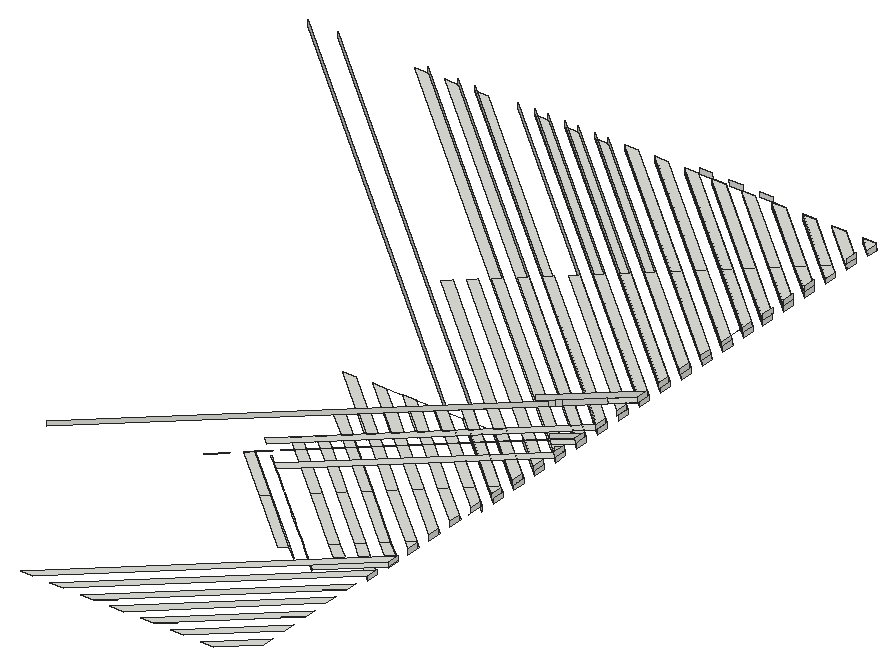
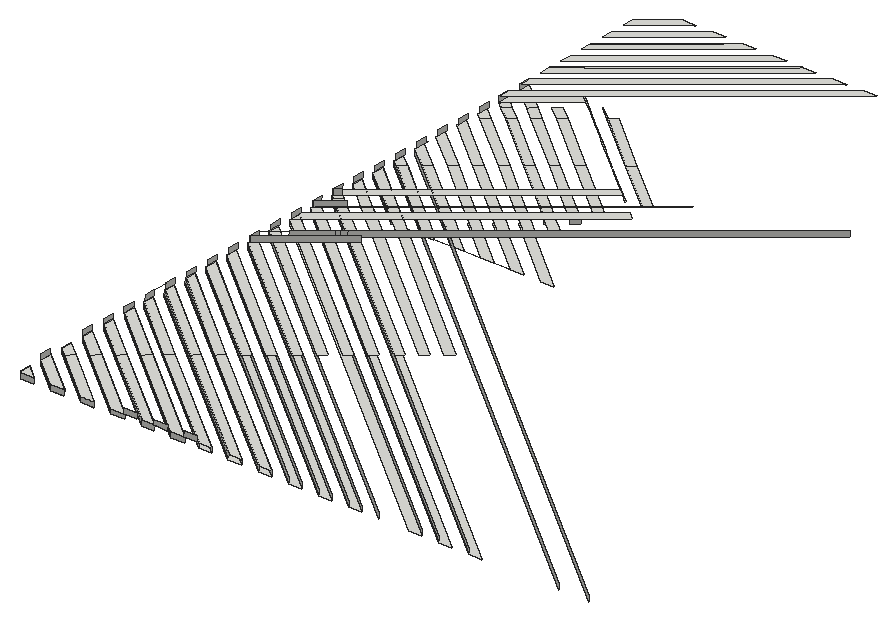
# SketchUp Ruby script. Lengths in inches.
U = 1.inch
M = Sketchup.active_model
def pt(a) = Geom::Point3d.new(a.map { |v| v * U })
def face(e, loops, mat)
  f = e.add_face(loops[0].map { |a| pt(a) })
  loops[1..].each { |l| e.add_face(l.map { |a| pt(a) }).erase! }
  f.material = f.back_material = mat if mat
  f
end
# faces: each face lists its corners as indices into pts; further lists are holes
def faces(e, pts, list, mat = nil) = list.each { |f| face(e, (f[0].is_a?(Array) ? f : [f]).map { |l| l.map { |i| pts[i] } }, mat) }
# xy, xz, yz: faces in a plane at the given z, y or x. An outline is a flat list of corners, or four numbers for a rectangle; further outlines are holes
def ring(l) = l.size == 4 ? [[l[0], l[1]], [l[2], l[1]], [l[2], l[3]], [l[0], l[3]]] : l.each_slice(2).to_a
def flat(e, list, mat, &to3) = list.each { |f| face(e, (f[0].is_a?(Array) ? f : [f]).map { |l| ring(l).map { |u, v| to3.(u, v) } }, mat) }
def xy(e, z, list, mat = nil) = flat(e, list, mat) { |x, y| [x, y, z] }
def xz(e, y, list, mat = nil) = flat(e, list, mat) { |x, z| [x, y, z] }
def yz(e, x, list, mat = nil) = flat(e, list, mat) { |y, z| [x, y, z] }
def lines(e, pts, list) = list.each { |a, b| e.add_line(pt(pts[a]), pt(pts[b])) }
# prism: a flat outline (further loops are holes) pulled along v
def prism(e, loops, v, mat = nil)
  f = face(e, loops, mat); d = Geom::Vector3d.new(v.map { |x| x * U })
  f.pushpull(f.normal.samedirection?(d) ? d.length : -d.length)
end
def box(e, o, s, mat = nil) = prism(e, [[o, [o[0] + s[0], o[1], o[2]], [o[0] + s[0], o[1] + s[1], o[2]], [o[0], o[1] + s[1], o[2]]]], [0, 0, s[2]], mat)
def at(x, y, z, deg = 0) = Geom::Transformation.translation(pt([x, y, z])) * Geom::Transformation.rotation(ORIGIN, Z_AXIS, deg.degrees)
def axes(o, x, y, z) = Geom::Transformation.new([*x, 0, *y, 0, *z, 0, *pt(o).to_a, 1])
def part(name) = M.definitions.add(name)
# library, detail: a bought-in or finely detailed component or shape, given as its bounding box
def library(name, o, s) = part(name).tap { |d| box(d.entities, o, s) }
def detail(e, o, s) = box(e.add_group.entities, o, s)
def put(e, d, t, mat = nil) = e.add_instance(d, t).tap { |i| i.material = mat if mat }
def group(e, t, mat = nil) = e.add_group.tap { |g| g.transformation = t; g.material = mat if mat }.entities
root = M.entities
yz(root,1888.28,[[651.23,111.967,653.518,112.048,653.496,113.075,651.207,112.994]])
yz(root,1888.281,[[635.202,111.398,637.555,111.482,637.532,112.509,635.179,112.425],[640.566,111.589,642.855,111.67,642.832,112.697,640.544,112.615],[635.305,112.459,637.658,112.543,637.636,113.57,635.282,113.486]])
yz(root,1888.282,[[624.538,111.02,624.515,112.047,626.869,112.131,626.891,111.104],[629.903,111.211,632.191,111.292,632.169,112.319,629.88,112.237],[624.642,112.081,626.995,112.165,626.972,113.192,624.619,113.108],[630.005,112.272,632.293,112.353,632.271,113.38,629.982,113.298]])
yz(root,1888.283,[[609.116,110.474,611.404,110.555,611.382,111.582,610.967,111.567,609.093,111.5],[614.414,110.661,616.767,110.745,616.745,111.772,616.332,111.757,614.392,111.688],[608.679,111.486,609.093,111.5,610.967,111.567,610.966,111.597,610.944,112.624,608.655,112.542,608.678,111.515],[613.979,111.674,614.392,111.688,616.332,111.757,616.331,111.787,616.309,112.814,613.956,112.73,613.978,111.703]])
yz(root,1888.284,[[598.452,110.096,600.741,110.177,600.718,111.204,598.43,111.122],[603.751,110.283,606.104,110.367,606.081,111.394,603.728,111.31],[598.014,111.137,600.303,111.219,600.28,112.245,597.992,112.164],[603.315,111.325,605.668,111.409,605.645,112.436,603.292,112.352]])
yz(root,1888.285,[[587.789,109.717,590.077,109.799,590.055,110.826,587.766,110.744],[593.088,109.905,595.441,109.989,595.418,111.016,593.065,110.932],[587.351,110.759,589.639,110.84,589.617,111.867,587.328,111.786],[592.651,110.947,595.004,111.031,594.982,112.058,592.629,111.974]])
yz(root,1888.286,[[571.761,109.149,574.114,109.233,574.091,110.26,573.49,110.238,571.738,110.176],[577.126,109.339,579.414,109.421,579.391,110.447,578.977,110.433,577.103,110.366],[571.324,110.191,571.813,110.208,573.489,110.268,573.677,110.275,573.655,111.302,571.302,111.218],[576.6875,110.381,578.976,110.462,578.953,111.489,576.665,111.408]])
yz(root,1888.287,[[561.097,108.771,563.45,108.855,563.428,109.882,563.042,109.868,561.075,109.798],[566.462,108.961,568.751,109.043,568.728,110.069,568.313,110.055,566.439,109.988],[560.662,109.783,561.075,109.798,563.042,109.868,563.019,110.924,562.991,110.923,560.638,110.84],[566.025,109.974,566.439,109.988,568.313,110.055,568.3125,110.084,568.29,111.111,566.001,111.03,566.024,110.003]])
yz(root,1888.288,[[549.998,109.405,549.997,109.435,549.975,110.462,552.328,110.545,552.351,109.519,552.351,109.489,550.411,109.42]])
yz(root,1888.289,[[534.038,108.84,534.449,108.854,536.323,108.921,536.322,108.95,536.3,109.977,534.015,109.896],[539.341,109.028,539.748,109.042,541.688,109.111,541.687,109.14,541.664,110.167,539.317,110.084]])
yz(root,1888.29,[[523.76,108.475,523.786,108.476,526.074,108.557,526.113,108.559,526.112,108.588,526.089,109.615,523.736,109.532,523.759,108.505],[529.084,108.664,529.123,108.665,529.122,108.695,529.084,108.694],[529.123,108.665,531.411,108.746,531.41,108.776,529.122,108.695],[529.122,108.695,531.41,108.776,531.388,109.803,529.099,109.722]])
p = [[1888.29,531.388,109.803],[1842.806,491.875,108.402],[1845.44,491.875,108.402],[1888.29,529.099,109.722],[1888.29,526.089,109.615],[1848.906,491.875,108.402],
  [1851.615,491.876,108.402],[1888.29,523.736,109.532],[1888.29,520.724,109.425],[1855.082,491.876,108.402],[1857.715,491.876,108.402],[1888.291,518.44,109.344],
  [1857.717,491.876,108.402],[1888.291,518.436,109.344],[1888.291,515.426,109.237],[1861.182,491.876,108.402],[1863.891,491.876,108.402],[1888.291,513.073,109.154],
  [1888.291,510.061,109.047],[1867.359,491.877,108.402],[1869.993,491.877,108.402],[1888.291,507.772,108.966],[1869.998,491.877,108.402],[1888.291,507.767,108.966],
  [1888.292,504.762,108.859],[1873.459,491.877,108.402],[1876.168,491.877,108.402],[1888.292,502.409,108.776],[1888.292,499.397,108.669],[1879.635,491.877,108.402],
  [1882.27,491.877,108.402],[1888.292,497.109,108.588],[1877.723,522.231,108.451],[1877.752,522.257,108.452],[1879.071,521.114,108.411],[1879.041,521.087,108.41],
  [1888.29,529.122,108.695],[1888.29,531.41,108.776],[1874.517,522.073,108.415],[1874.507,522.064,108.415],[1871.456,524.716,108.509],[1871.465,524.724,108.509],
  [1874.922,524.71,108.539],[1874.896,524.687,108.538],[1857.84,534.204,108.845],[1859.189,535.376,108.887],[1870.111,523.547,108.468],[1888.29,526.074,108.557],
  [1888.29,523.786,108.476],[1882.388,528.911,108.658],[1883.706,530.056,108.698],[1859.194,535.38,108.887],[1871.831,527.39,108.634],[1871.807,527.369,108.633],
  [1865.325,572.707,110.211],[1870.153,568.514,110.062],[1873.198,565.869,109.968],[1883.742,556.712,109.643],[1888.288,552.764,109.503],[1888.288,552.787,108.477],
  [1870.153,568.537,109.035],[1864.425,573.511,109.211],[1771.79,653.962,112.063],[1771.79,653.939,113.09],[1834.633,599.362,111.155],[1853.473,554.046,108.521],
  [1854.79,555.191,108.562],[1854.79,555.168,109.589],[1853.473,554.024,109.548],[1880.655,527.405,108.604],[1879.3,526.229,108.563],[1876.248,528.879,108.657],
  [1877.602,530.056,108.698],[1870.096,528.893,108.687],[1870.074,528.874,108.686],[1888.288,555.799,108.583],[1888.288,555.776,109.61],[1885.476,558.218,109.697],
  [1874.932,567.375,110.021],[1871.886,570.02,110.115],[1871.886,570.043,109.088],[1873.204,571.187,109.129],[1888.287,558.087,108.664],[1888.287,557.65,109.677],
  [1888.287,558.064,109.691],[1856.523,556.696,108.615],[1857.877,557.872,108.657],[1857.877,557.85,109.684],[1856.523,556.673,109.642],[1863.977,539.537,109.035],
  [1865.331,540.713,109.076],[1868.777,530.036,108.727],[1868.757,530.018,108.727],[1879.336,531.562,108.752],[1880.653,532.707,108.792],[1885.438,531.561,108.752],
  [1886.778,532.725,108.793],[1888.29,531.411,108.746],[1888.29,529.123,108.665],[1888.29,529.084,108.664],[1867.042,531.541,108.781],[1867.023,531.524,108.78],
  [1888.29,531.437,108.747],[1886.792,532.737,108.793],[1868.376,575.358,110.304],[1873.204,571.164,110.156],[1876.249,568.52,110.062],[1886.793,559.363,109.737],
  [1870.527,573.512,109.211],[1777.893,653.962,112.063],[1777.893,653.94,113.09],[1837.684,602.012,111.249],[1859.611,559.379,108.71],[1843.339,573.51,109.211],
  [1845.974,573.51,109.211],[1860.928,560.523,108.751],[1877.569,583.314,111.644],[1817.09,530.779,109.781],[1817.087,530.804,108.755],[1876.29,582.231,110.578],
  [1877.205,583.027,110.606],[1877.566,583.339,110.617],[1865.686,532.716,108.822],[1865.668,532.701,108.822],[1867.065,542.22,109.13],[1868.382,543.364,109.17],
  [1882.386,534.212,108.846],[1883.727,535.377,108.887],[1863.951,534.219,108.876],[1863.935,534.205,108.875],[1883.74,535.388,108.887],[1848.646,544.539,109.212],
  [1847.293,543.363,109.17],[1870.114,544.869,109.224],[1871.461,546.04,109.265],[1875.88,573.512,109.211],[1876.701,573.512,109.211],[1888.287,563.45,108.855],
  [1888.287,561.097,108.771],[1874.936,572.692,109.182],[1888.287,561.075,109.798],[1877.982,570.025,110.115],[1874.936,572.67,110.209],[1862.66,562.028,108.804],
  [1849.439,573.51,109.211],[1852.148,573.511,109.211],[1864.015,563.205,108.846],[1862.633,535.362,108.916],[1862.618,535.35,108.916],[1885.474,536.895,108.941],
  [1886.791,538.039,108.981],[1888.289,536.738,108.935],[1888.289,536.323,108.921],[1888.289,534.449,108.854],[1857.807,539.546,109.065],[1857.797,539.537,109.064],
  [1848.647,544.54,109.212],[1871.468,546.046,109.265],[1873.202,547.552,109.319],[1874.519,548.697,109.359],[1888.287,563.428,109.882],[1876.291,573.869,109.224],
  [1876.291,573.846,110.251],[1879.336,571.201,110.157],[1865.749,564.711,108.899],[1855.616,573.511,109.211],[1858.25,573.511,109.211],[1867.066,565.855,108.94],
  [1844.243,540.714,109.076],[1842.51,539.208,109.023],[1884.163,575.394,110.335],[1888.286,578.976,110.462],[1888.286,578.977,110.433],[1887.207,578.04,110.4],
  [1885.474,576.534,110.346],[1884.119,575.357,110.304],[1882.387,573.852,110.251],[1881.07,572.707,110.211],[1871.844,564.692,109.926],[1870.111,563.187,109.873],
  [1868.794,562.043,109.832],[1867.061,560.537,109.779],[1865.706,559.36,109.737],[1863.974,557.855,109.684],[1862.656,556.711,109.643],[1860.923,555.205,109.59],
  [1860.921,555.203,109.59],[1859.569,554.028,109.548],[1857.836,552.523,109.495],[1856.519,551.378,109.454],[1854.785,549.872,109.401],[1853.431,548.696,109.359],
  [1851.698,547.19,109.306],[1845.561,541.858,109.117],[1876.251,550.202,109.413],[1877.605,551.379,109.454],[1888.289,542.101,109.125],[1888.289,541.688,109.111],
  [1888.289,539.748,109.042],[1888.287,566.462,108.961],[1888.287,566.439,109.988],[1880.169,573.49,110.238],[1880.169,573.512,109.211],[1868.798,567.36,108.993],
  [1861.716,573.511,109.211],[1856.488,540.689,109.105],[1856.479,540.681,109.105],[1854.753,542.193,109.158],[1854.745,542.187,109.158],[1867.892,573.512,109.211],
  [1888.286,571.761,109.149],[1888.286,571.738,110.176],[1886.269,573.49,110.238],[1886.269,573.513,109.211],[1793.635,653.963,112.064],[1796.344,653.964,112.064],
  [1872.056,588.21,109.732],[1884.849,577.099,109.338],[1888.286,574.114,109.233],[1853.391,543.363,109.2],[1853.397,543.368,109.2],[1888.286,571.324,110.191],
  [1884.961,570.789,110.172],[1887.213,572.745,110.242],[1888.286,571.813,110.208],[1851.662,544.872,109.253],[1851.658,544.868,109.253],[1888.289,544.698,109.218],
  [1888.289,544.697,109.247],[1888.289,544.675,110.274],[1888.288,546.963,110.355],[1888.288,546.986,109.328],[1888.288,546.986,109.299],[1888.288,545.113,109.232],
  [1879.339,552.885,109.508],[1880.656,554.03,109.548],[1888.288,547.401,109.313],[1887.623,574.667,110.28],[1888.286,574.091,110.26],[1796.344,653.941,113.09],
  [1846.909,610.026,111.534],[1888.286,581.988,110.569],[1848.608,547.519,109.347],[1847.252,548.695,109.389],[1888.285,584.341,110.653],[1802.446,653.964,112.064],
  [1888.286,579.414,109.421],[1888.286,577.126,109.339],[1884.162,580.707,109.466],[1881.944,582.633,109.535],[1799.811,653.964,112.064],[1888.286,577.103,110.366],
  [1884.162,580.684,110.493],[1851.739,552.518,109.495],[1850.385,551.341,109.453],[1882.388,555.535,109.602],[1888.288,552.351,109.489],[1888.288,550.411,109.42],
  [1849.96,612.677,111.628],[1885.479,581.829,110.534],[1888.286,579.391,110.447],[1802.446,653.941,113.09],[1888.285,584.777,109.611],[1888.286,582.424,109.527],
  [1887.212,583.356,109.56],[1881.944,587.932,109.723],[1805.911,653.964,112.064],[1808.62,653.964,112.064],[1888.286,582.401,110.554],[1887.212,583.334,110.587],
  [1888.285,584.754,110.638],[1888.285,584.266,110.62],[1888.288,555.361,109.596],[1888.288,555.361,109.625],[1888.288,555.338,110.652],[1888.287,557.626,110.733],
  [1888.287,557.649,109.706],[1853.048,562.043,109.832],[1851.694,560.867,109.791],[1860.928,560.5,109.778],[1859.611,559.356,109.737],[1886.205,584.208,110.618],
  [1885.436,584.876,110.642],[1851.692,614.182,111.681],[1805.911,653.941,113.09],[1856.099,564.694,109.926],[1854.782,563.549,109.886],[1864.015,563.182,109.873],
  [1862.66,562.005,109.831],[1888.287,563.042,109.868],[1859.187,567.375,110.021],[1857.832,566.199,109.98],[1867.066,565.832,109.967],[1865.749,564.688,109.926],
  [1856.097,618.009,111.817],[1888.285,590.055,110.826],[1888.285,590.077,109.799],[1814.723,653.965,112.064],[1814.723,653.942,113.09],[1862.237,570.026,110.115],
  [1860.92,568.881,110.075],[1868.798,567.337,110.02],[1888.285,593.088,109.905],[1818.188,653.965,112.064],[1820.897,653.965,112.064],[1888.285,595.441,109.989],
  [1888.285,593.065,110.932],[1857.83,619.514,111.87],[1818.188,653.942,113.091],[1888.287,568.313,110.055],[1888.287,568.728,110.069],[1863.97,571.531,110.169],
  [1859.184,620.691,111.912],[1888.285,595.418,111.016],[1820.897,653.942,113.091],[1867.058,574.213,110.264],[1824.365,653.965,112.064],[1888.284,598.452,110.096],
  [1888.284,598.43,111.122],[1860.918,622.197,111.965],[1824.365,653.943,113.091],[1826.999,653.965,112.064],[1888.284,600.741,110.177],[1888.286,573.49,110.238],
  [1888.286,573.489,110.268],[1888.286,573.677,110.275],[1843.822,607.345,111.438],[1842.505,606.2,111.398],[1871.463,578.039,110.4],[1870.108,576.863,110.358],
  [1888.286,573.655,111.302],[1887.213,572.722,111.268],[1826.999,653.943,113.091],[1862.235,623.341,112.006],[1888.284,600.718,111.204],[1888.286,576.6875,110.381],
  [1885.48,574.25,110.295],[1845.554,608.85,111.492],[1888.286,578.953,111.489],[1884.163,575.372,111.362],[1830.465,653.966,112.064],[1888.284,603.751,110.283],
  [1888.284,603.728,111.31],[1863.967,624.847,112.059],[1830.465,653.943,113.091],[1833.174,653.966,112.064],[1888.284,606.104,110.367],[1839.417,603.517,111.303],
  [1840.771,604.694,111.345],[1865.322,626.023,112.101],[1888.284,606.081,111.394],[1833.174,653.943,113.091],[1848.642,611.532,111.587],[1888.283,609.116,110.474],
  [1836.641,653.966,112.064],[1839.276,653.966,112.064],[1888.283,611.404,110.555],[1888.283,609.093,111.5],[1867.055,627.529,112.154],[1836.641,653.943,113.091],
  [1888.286,581.965,111.596],[1888.285,584.318,111.68],[1874.935,583.408,110.62],[1888.285,595.004,111.031],[1888.285,592.651,110.947],[1884.605,589.454,110.834],
  [1879.141,584.708,110.666],[1878.444,584.102,110.644],[1853.046,615.359,111.723],[1878.447,584.077,111.671],[1874.935,583.385,111.646],[1888.285,594.982,112.058],
  [1879.144,584.682,111.692],[1868.373,628.674,112.195],[1888.283,611.382,111.582],[1839.276,653.943,113.091],[1884.608,589.429,111.861],[1854.78,616.865,111.776],
  [1888.285,587.766,110.744],[1888.283,614.414,110.661],[1842.741,653.966,112.064],[1845.45,653.966,112.064],[1888.283,616.767,110.745],[1888.283,614.392,111.688],
  [1870.105,630.179,112.248],[1842.741,653.944,113.091],[1871.46,631.355,112.29],[1888.283,616.745,111.772],[1845.45,653.944,113.091],[1888.283,619.779,110.852],
  [1848.918,653.967,112.064],[1851.553,653.967,112.064],[1888.282,622.068,110.933],[1888.283,619.757,111.879],[1873.193,632.862,112.343],[1848.918,653.944,113.091],
  [1888.282,622.045,111.96],[1874.51,634.006,112.384],[1851.553,653.944,113.091],[1888.282,626.891,111.104],[1888.282,624.538,111.02],[1854.397,653.967,112.064],
  [1857.106,653.967,112.064],[1888.282,624.515,112.047],[1875.932,635.241,112.428],[1854.397,653.944,113.091],[1877.287,636.418,112.469],[1888.282,626.869,112.131],
  [1857.106,653.945,113.091],[1860.573,653.967,112.064],[1863.208,653.968,112.064],[1888.282,632.191,111.292],[1888.282,629.903,111.211],[1888.282,629.88,112.237],
  [1879.02,637.924,112.523],[1860.573,653.945,113.091],[1880.337,639.068,112.563],[1888.282,632.169,112.319],[1863.208,653.945,113.091],[1866.673,653.968,112.064],
  [1869.382,653.968,112.064],[1888.281,637.555,111.482],[1888.281,635.202,111.398],[1888.281,635.179,112.425],[1882.07,640.574,112.617],[1866.673,653.945,113.091],
  [1888.283,610.967,111.567],[1883.424,641.75,112.658],[1888.281,637.532,112.509],[1869.382,653.945,113.091],[1872.85,653.968,112.064],[1888.281,640.566,111.589],
  [1888.281,640.544,112.615],[1885.158,643.256,112.712],[1872.85,653.945,113.091],[1888.281,642.855,111.67],[1875.484,653.968,112.064],[1888.283,616.332,111.757],
  [1875.484,653.946,113.091],[1886.475,644.401,112.752],[1888.281,642.832,112.697],[1878.95,653.968,112.064],[1888.281,645.865,111.776],[1888.281,645.842,112.803],
  [1888.208,645.906,112.806],[1878.95,653.946,113.091],[1888.281,645.969,112.808],[1888.28,648.218,111.86],[1888.28,648.195,112.887],[1881.659,653.969,112.064],
  [1888.283,619.341,111.894],[1888.282,621.63,111.975],[1888.282,621.607,113.002],[1888.283,619.319,112.92],[1881.659,653.946,113.091],[1888.28,653.518,112.048],
  [1888.28,651.23,111.967],[1885.126,653.969,112.064],[1887.761,653.969,112.064],[1888.28,651.207,112.994],[1885.126,653.946,113.091],[1888.28,653.496,113.075],
  [1887.761,653.946,113.091],[1854.459,653.944,113.091],[1860.634,653.945,113.091],[1866.736,653.945,113.091],[1885.187,653.946,113.091],[1888.28,648.322,112.921],
  [1888.28,648.299,113.948],[1888.281,645.946,113.864],[1888.28,648.322,112.891],[1851.825,653.921,114.147],[1854.459,653.921,114.147],[1854.459,653.944,113.12],
  [1851.825,653.944,113.091],[1851.825,653.944,113.12],[1857.925,653.921,114.147],[1860.634,653.922,114.147],[1860.634,653.944,113.12],[1857.925,653.945,113.091],
  [1857.925,653.944,113.12],[1864.101,653.922,114.147],[1866.736,653.922,114.147],[1866.736,653.944,113.12],[1864.101,653.945,113.091],[1864.101,653.944,113.12],
  [1873.992,573.512,109.211],[1884.608,589.452,110.834],[1884.605,589.455,110.804],[1888.283,616.309,112.814],[1888.285,592.629,111.974],[1888.288,549.244,109.379],
  [1888.288,549.998,109.405],[1888.285,592.652,110.918],[1885.187,653.946,113.12]]
faces(root,p,[[0,1,2,3],[4,5,6,7],[8,9,10,11],[11,10,12,13],[14,15,16,17],[18,19,20,21],[20,22,23,21],[24,25,26,27],
  [28,29,30,31],[32,33,34,35],[36,34,33,37],[38,39,40,41],[42,33,32,43],[44,45,40,46],[47,48,49,50],[41,40,45,51],
  [52,42,43,53],[54,55,56,57,58,59,60,61,62,63,64],[65,66,67,68],[69,70,71,72],[73,52,53,74],[75,76,77,78,79,80],[80,81,82,75],[83,76,75,82,84],
  [85,86,87,88],[72,71,89,90],[91,73,74,92],[50,49,93,94],[95,96,97,98,99],[100,91,92,101],[102,97,96,103],[104,105,106,107,84,82,81,108,109,110,111],
  [112,113,114,115],[116,117,118,119,120,121],[122,100,101,123],[94,93,124,125],[126,127,96,95],[128,122,123,129],[103,96,127,130],[44,45,131,132],
  [133,134,127,126],[135,136,137,138,139],[138,140,141,142,139],[143,144,145,146],[147,128,129,148],[149,150,151,152,153],[154,147,148,155],[156,131,45,51],
  [130,127,134,157],[158,159,150,149],[160,137,136,161,162,163],[164,165,166,167],[168,169,170,171,172,173,174,175,176,177,163,141,106,78,56,178,179,180,181,182,183,184,185,186,187,188,189,190,191,192,156,131,132,193],[190,191,89,90],[194,195,196,197,198],[199,200,177,201,202],
  [203,204,61,60],[205,154,155,206],[207,205,206,208],[188,189,124,125],[80,209,108,81],[210,211,212,213],[210,213,214,215,216,217,218],[219,220,207,208],
  [221,207,220,222,223,224],[225,220,219,226],[227,228,229,230,231,232,233],[133,134,186,187],[234,235,236,232,233],[135,161,162,142,139],[161,136,135],[174,237,238,218,217,216,215,239,240],
  [185,186,134,157],[241,242,243,244],[158,159,183,184],[245,246,247,248,249,250],[247,251,173,252,248],[253,254,191,190],[194,195,181,182],[255,57,58,256,257],
  [258,259,260,246,245,261],[67,68,189,188],[234,235,179,180],[187,186,87,88],[262,263,264,265,266,267],[264,263,268,269],[262,270,271,268,263],[185,87,186],
  [272,273,274,275,276,83,76],[255,57,56,178],[77,107,84,83,76],[87,277,278,88],[184,183,279,280],[265,264,269,281,282,283,284,266],[77,107,106,78],[279,285,286,280],
  [182,181,287,288],[289,160,163,141,140],[287,290,291,288],[180,179,292,293],[294,295,296,297,298],[292,299,300,293],[178,56,55,301],[302,303,304,305],
  [303,302,306,307,308],[176,177,200,309,310],[55,54,311,301],[78,106,105,79],[312,313,305,304,314],[105,104,315,79],[141,163,162,142],[316,317,318,319,320],
  [317,316,321,322],[323,238,237,212,211],[324,224,223,325],[326,327,201,177,176],[162,328,329,142],[330,325,223,331],[237,174,175,212],[332,333,334,322,321],
  [171,335,336,170],[337,175,174,240],[338,171,170,339],[340,341,342,343,344],[341,340,345,346],[347,329,328,348],[172,173,251],[259,252,173,172,260],
  [349,350,346,345,351],[258,352,252,259],[353,354,355,356],[354,353,357,358,359],[360,241,244,361],[121,120,119,362,363,364,365,366,367],[269,268,271],[368,283,282,281,269,271,270],
  [367,369,116,121],[363,362,370,371],[372,369,367,366],[373,374,356,355,375],[376,372,366,365],[294,377,378,295],[379,380,381,382],[380,379,383,384,385],
  [386,387,382,381,388],[313,312,307,306],[389,390,391,392],[390,389,393,394,395],[392,396,393,389],[397,396,392,391,398],[399,400,401,402],[401,400,403,404,405],
  [334,333,319,318],[406,407,399,402,408],[409,410,411,412],[409,412,413,414,415],[350,349,343,342],[416,417,411,410,418],[419,420,421,422],[419,422,423,424,425],
  [374,373,358,357,426],[427,428,421,420,429],[430,431,432,433,434],[435,431,430,436],[387,386,384,383,437],[438,439,440,435,436],[441,442,443,444,445],[446,443,442,447,448],
  [447,442,441,449],[450,451,452,453],[396,397,394,393],[454,448,447,449],[407,406,404,403],[455,456,457,458],[456,459,460,457],[461,455,458,462],
  [402,401,405,463,408],[410,409,415,464,418],[420,419,425,465,429],[436,430,434,438],[449,441,445,454],[462,458,457,460,466],[359,358,373,375],[417,416,414,413],
  [385,384,386,388],[395,394,397,398],[405,404,406,408,463],[428,427,424,423],[415,414,416,418,464],[440,439,433,432],[425,424,427,429,465],[434,433,439,438],
  [443,446,444],[445,444,446,448,454],[467,468,469,446,448,470],[460,459,461,462,466],[471,472,473,463,405,474,475],[476,477,478,464,415,479,480],[481,482,483,465,425,484,485]])
lines(root,p,[[286,277],[209,61],[486,108],[204,166],[165,145],[300,290],[364,487],[329,104],[365,488],[323,324],[489,453],[315,54],
  [376,490],[491,492],[311,299],[493,364],[291,285],[466,494]])
